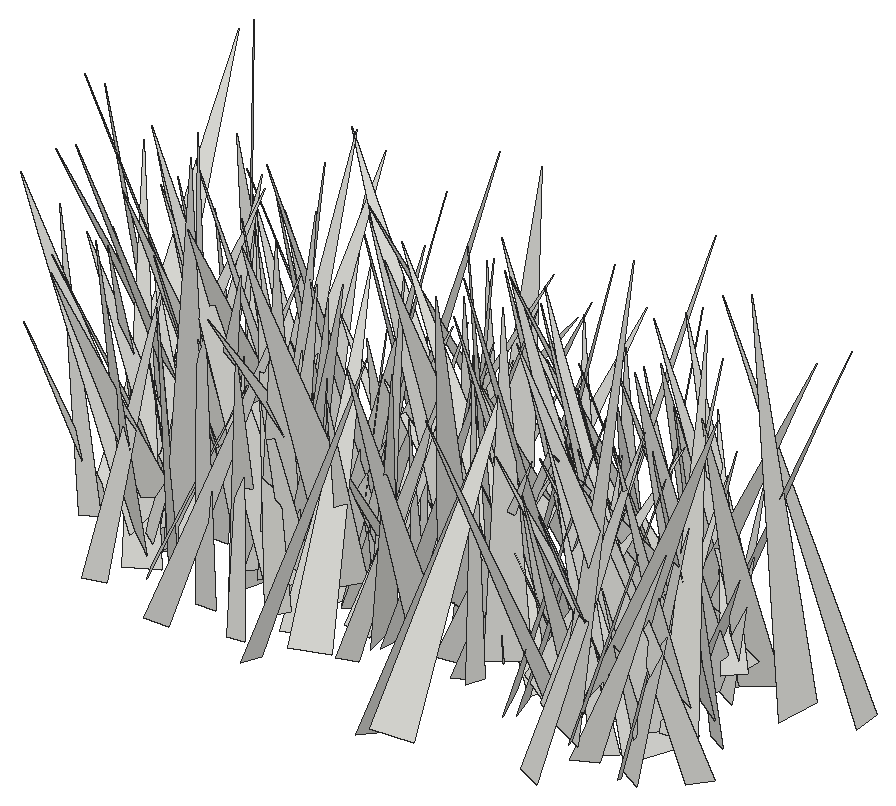
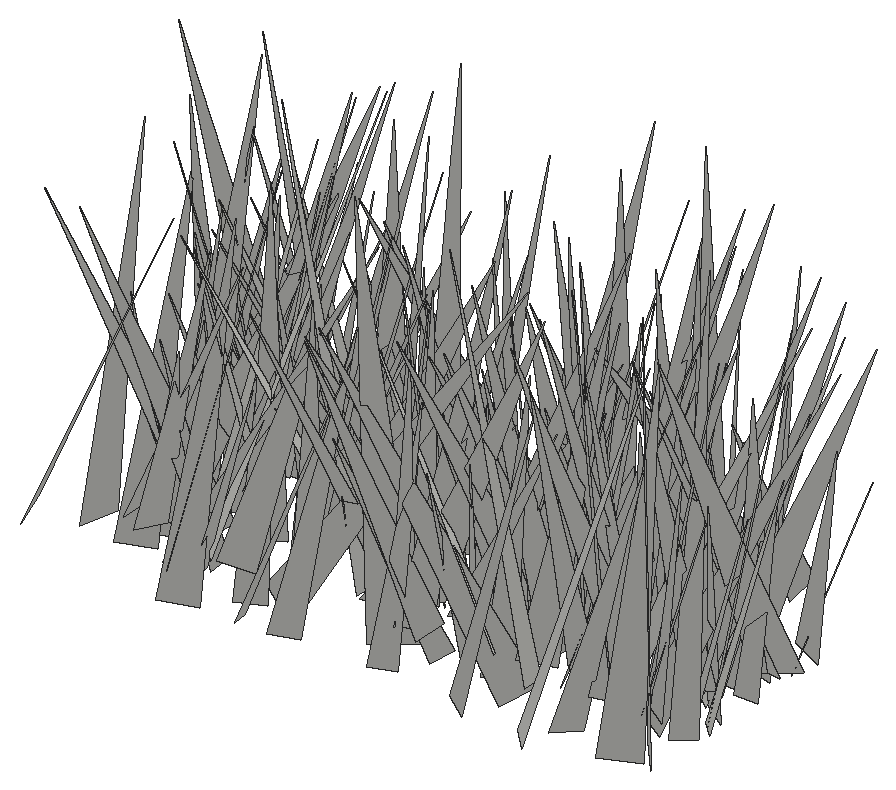
# SketchUp Ruby script. Lengths in inches.
U = 1.inch
M = Sketchup.active_model
def pt(a) = Geom::Point3d.new(a.map { |v| v * U })
def face(e, loops, mat)
  f = e.add_face(loops[0].map { |a| pt(a) })
  loops[1..].each { |l| e.add_face(l.map { |a| pt(a) }).erase! }
  f.material = f.back_material = mat if mat
  f
end
# faces: each face lists its corners as indices into pts; further lists are holes
def faces(e, pts, list, mat = nil) = list.each { |f| face(e, (f[0].is_a?(Array) ? f : [f]).map { |l| l.map { |i| pts[i] } }, mat) }
# xy, xz, yz: faces in a plane at the given z, y or x. An outline is a flat list of corners, or four numbers for a rectangle; further outlines are holes
def ring(l) = l.size == 4 ? [[l[0], l[1]], [l[2], l[1]], [l[2], l[3]], [l[0], l[3]]] : l.each_slice(2).to_a
def flat(e, list, mat, &to3) = list.each { |f| face(e, (f[0].is_a?(Array) ? f : [f]).map { |l| ring(l).map { |u, v| to3.(u, v) } }, mat) }
def xy(e, z, list, mat = nil) = flat(e, list, mat) { |x, y| [x, y, z] }
def xz(e, y, list, mat = nil) = flat(e, list, mat) { |x, z| [x, y, z] }
def yz(e, x, list, mat = nil) = flat(e, list, mat) { |y, z| [x, y, z] }
def lines(e, pts, list) = list.each { |a, b| e.add_line(pt(pts[a]), pt(pts[b])) }
# prism: a flat outline (further loops are holes) pulled along v
def prism(e, loops, v, mat = nil)
  f = face(e, loops, mat); d = Geom::Vector3d.new(v.map { |x| x * U })
  f.pushpull(f.normal.samedirection?(d) ? d.length : -d.length)
end
def box(e, o, s, mat = nil) = prism(e, [[o, [o[0] + s[0], o[1], o[2]], [o[0] + s[0], o[1] + s[1], o[2]], [o[0], o[1] + s[1], o[2]]]], [0, 0, s[2]], mat)
def at(x, y, z, deg = 0) = Geom::Transformation.translation(pt([x, y, z])) * Geom::Transformation.rotation(ORIGIN, Z_AXIS, deg.degrees)
def axes(o, x, y, z) = Geom::Transformation.new([*x, 0, *y, 0, *z, 0, *pt(o).to_a, 1])
def part(name) = M.definitions.add(name)
# library, detail: a bought-in or finely detailed component or shape, given as its bounding box
def library(name, o, s) = part(name).tap { |d| box(d.entities, o, s) }
def detail(e, o, s) = box(e.add_group.entities, o, s)
def put(e, d, t, mat = nil) = e.add_instance(d, t).tap { |i| i.material = mat if mat }
def group(e, t, mat = nil) = e.add_group.tap { |g| g.transformation = t; g.material = mat if mat }.entities
root = M.entities
c1 = part("fur_instance\#9")
p = [[0.8125,0,1.79],[0.67,-0.02,1.48],[0,-0.11,0],[0,0.11,0]]
faces(c1.entities,p,[[0,1,2,3]])
put(root,c1,axes([77.6,147.16,-27.1],[6.21031,-0.46369,2.15458],[0.49806,-5.98034,-2.72263],[-2.14689,-2.7287,5.60092]))
put(root,c1,axes([84.37,145.48,-27.1],[-1.75901,-5.06572,0.78099],[-4.97011,1.48393,-1.5689],[-1.25276,1.22556,5.12778]))
put(root,c1,axes([66.86,146.18,-28.22],[-2.48382,-6.27006,1.58629],[-6.2632,2.75568,1.08533],[1.61318,1.04494,6.65621]))
put(root,c1,axes([80.48,142.09,-28.22],[-3.2571,5.60614,0.8435],[5.30317,3.35677,-1.83235],[2.00417,0.22864,6.21933]))
put(root,c1,axes([85.58,147.03,-27.1],[-2.3415,-4.6423,0.1365],[-4.37976,2.25803,1.66471],[1.54509,-0.63449,4.92568]))
put(root,c1,axes([73.91,143.17,-28.22],[5.46763,0.70402,1.09334],[0.38726,-5.3924,1.5356],[-1.2414,1.41859,5.29457]))
put(root,c1,axes([69.07,144.02,-27.1],[3.47844,1.93474,0.04271],[1.93521,-3.47755,-0.07868],[0.00093,-0.08952,3.97952]))
put(root,c1,axes([67.8125,147.34,-28.22],[2.22572,-6.24997,0.53761],[-6.03536,-2.28904,-1.62473],[-1.71046,-0.05581,6.43243]))
put(root,c1,axes([86.3,144.63,-28.22],[3.70527,-2.55389,0.75103],[-2.66189,-3.54115,1.0909],[0.02774,1.32414,4.36593]))
put(root,c1,axes([68.62,145.87,-28.22],[4.97052,1.68586,2.30908],[2.28367,-5.12743,-1.17229],[-1.72012,-1.9358,5.11604]))
put(root,c1,axes([85.55,142.73,-28.22],[2.91229,5.1803,0.24137],[5.15397,-2.92189,0.52374],[-0.57474,0.04729,5.91968]))
put(root,c1,axes([84.36,146.93,-28.22],[5.01646,-0.03484,2.02413],[0.79085,-4.94522,-2.0451],[-1.86357,-2.19241,4.58078]))
put(root,c1,axes([71.29,141.59,-27.1],[-5.44791,2.04028,1.98238],[0.64646,5.0587,-3.42987],[2.77031,2.83181,4.69878]))
put(root,c1,axes([68.04,142.5,-27.1],[-4.70225,1.57903,0.9136],[0.9953,4.33742,-2.37389],[1.52885,2.03289,4.35536]))
put(root,c1,axes([79.77,141.68,-28.22],[7.02675,2.35333,1.41841],[1.60681,-6.67867,3.12071],[-2.22895,2.60433,6.72121]))
put(root,c1,axes([84.85,144.68,-27.1],[2.54446,5.11145,1.43196],[5.2695,-2.24073,-1.36501],[0.64019,-1.87187,5.54418]))
put(root,c1,axes([72.7,143.875,-28.22],[0.97276,4.45119,0.9772],[4.35496,-1.20232,1.14148],[-1.3425,-0.67498,4.41093]))
put(root,c1,axes([70.92,146.67,-28.22],[4.90376,-2.85552,0.72078],[-2.73926,-4.93651,-0.92072],[-1.08166,-0.44414,5.59939]))
put(root,c1,axes([73.96,148.32,-27.1],[5.79186,-5.56058,1.06137],[-5.14067,-5.80215,-2.34538],[-2.37068,-1.00358,7.67886]))
put(root,c1,axes([88.27,146.18,-27.1],[1.0703,-6.74535,2.51722],[-6.58595,-1.94546,-2.41292],[-2.90886,1.9228,6.3893]))
put(root,c1,axes([68.65,146.46,-27.1],[7.59105,-2.36712,2.02897],[-2.18853,-7.84946,-0.96967],[-2.22043,-0.35586,7.89221]))
put(root,c1,axes([85.88,146.02,-27.1],[6.5822,-3.48627,0.04021],[-3.46978,-6.5418,0.80411],[0.34104,0.72931,7.40492]))
put(root,c1,axes([76.27,146.98,-28.22],[6.47505,-0.26988,1.20187],[0.07267,-6.33614,-1.81428],[-1.22965,-1.79557,6.22153]))
put(root,c1,axes([72.45,146.51,-27.1],[5.8288,-3.89293,1.62458],[-3.86791,-6.0381,-0.59132],[-1.68328,0.3943,6.98428]))
put(root,c1,axes([71.9,143.36,-27.1],[2.76553,6.92914,2.18566],[6.51494,-3.40021,2.53621],[-3.21647,-0.92942,7.01632]))
put(root,c1,axes([86.98,147.06,-28.22],[-5.50457,-1.9976,0.13924],[-1.94432,5.42927,1.02602],[0.47897,-0.91798,5.76524]))
put(root,c1,axes([86.59,145.36,-28.22],[0.57769,-3.84784,2.16026],[-4.16363,-1.197,-1.01866],[-1.46176,1.88882,3.75525]))
put(root,c1,axes([86.07,144,-27.1],[3.67219,7.15908,2.03524],[7.27938,-3.92759,0.68132],[-1.55086,-1.48365,8.01705]))
put(root,c1,axes([67.41,146.14,-27.1],[-3.27496,5.22829,1.96451],[5.47571,2.5569,2.32348],[-1.10043,-2.83671,5.71505]))
put(root,c1,axes([86.4,143.85,-27.1],[4.4489,2.71988,0.66857],[2.4928,-4.41728,1.38241],[-1.27698,0.85286,5.02786]))
put(root,c1,axes([70.7,148.35,-27.1],[0.98136,-7.62341,0.77855],[-7.49654,-1.11781,-1.49599],[-1.58884,0.56543,7.53933]))
put(root,c1,axes([78.21,148.41,-27.1],[0.34985,-8.1007,0.677],[-7.9597,-0.20383,1.67442],[1.6501,0.73429,7.93347]))
put(root,c1,axes([73.08,146.07,-27.1],[-8.06314,0.9505,0.88883],[1.02226,8.07835,0.63476],[0.80526,-0.7379,8.09412]))
put(root,c1,axes([88.92,146.52,-27.1],[-1.01611,-5.1437,1.43202],[-5.3112,0.8243,-0.80778],[-0.54728,1.55038,5.1805]))
put(root,c1,axes([73.09,147,-28.22],[3.60801,-2.69307,1.35493],[-2.4926,-3.85347,-1.02171],[-1.69571,-0.06573,4.3848]))
put(root,c1,axes([87.72,145.82,-27.1],[-7.02647,-2.17808,1.10616],[-2.29777,7.03636,-0.74079],[0.82938,1.04138,7.31892]))
put(root,c1,axes([64.94,146.83,-27.1],[-3.14416,-1.79317,0.28571],[-1.75542,3.14785,0.43854],[0.46429,-0.24163,3.59289]))
put(root,c1,axes([82.13,146.03,-28.22],[6.04949,2.12455,0.78775],[2.22415,-5.99674,-0.90711],[-0.43293,-1.1207,6.34722]))
put(root,c1,axes([90.05,145.83,-28.22],[-1.48445,-5.73193,2.26963],[-5.6541,0.33538,-2.85107],[-2.45713,2.69116,5.18942]))
put(root,c1,axes([67.28,148.54,-28.22],[-4.43936,-4.76816,0.23664],[-4.66276,4.39992,1.18262],[1.02469,-0.63608,6.40661]))
put(root,c1,axes([82.59,146.125,-28.22],[4.18181,1.0835,0.53294],[1.13424,-4.18373,-0.39425],[-0.41412,-0.51766,4.30187]))
put(root,c1,axes([81.59,146.6,-27.1],[4.24659,-4.94069,2.32668],[-5.22174,-4.53655,-0.10277],[-1.59916,1.69313,6.51409]))
put(root,c1,axes([73.99,144.41,-27.1],[-6.21207,0.31771,0.7174],[0.09871,5.99609,-1.80072],[0.77837,1.77522,5.95384]))
put(root,c1,axes([72.21,147.16,-28.22],[-7.46338,-1.41905,1.28497],[-1.31215,7.55774,0.72509],[1.39396,-0.48353,7.56241]))
put(root,c1,axes([87.75,146.16,-28.22],[-6.89397,4.20656,1.53795],[4.42912,6.82252,1.19307],[0.66584,-1.82904,7.9874]))
put(root,c1,axes([81.63,144.92,-27.1],[-5.20455,-0.25594,1.25726],[-0.61037,5.11409,-1.48563],[1.12857,1.58561,4.99457]))
put(root,c1,axes([83.66,147.67,-27.1],[-3.27464,-6.78559,1.40651],[-6.92909,3.22889,-0.5548],[0.10135,1.50857,7.51397]))
put(root,c1,axes([86.16,147.91,-28.22],[-3.67064,-4.64361,1.03864],[-4.58105,3.8034,0.81465],[1.28682,0.29416,5.86285]))
put(root,c1,axes([74.65,147.45,-27.1],[2.8154,-3.04723,0.70248],[-2.99803,-2.89898,-0.55973],[-0.88933,0.126,4.11081]))
put(root,c1,axes([72.54,151.18,-28.22],[-6.33754,-5.19611,0.8236],[-4.02771,5.62162,4.47406],[3.3846,-3.03975,6.86635]))
put(root,c1,axes([86.71,146.34,-27.1],[-8.26176,0.40654,0.83522],[0.41692,8.30295,0.08258],[0.83009,-0.12394,8.27135]))
put(root,c1,axes([72.48,147.22,-27.1],[6.13982,-1.63324,0.91897],[-1.58888,-6.20592,-0.4139],[-0.99371,-0.16841,6.33984]))
put(root,c1,axes([68.72,149.125,-28.22],[-3.15588,-6.30761,0.73503],[-6.08642,3.23856,1.65924],[1.81157,-0.10755,6.85511]))
put(root,c1,axes([78.95,147.05,-28.22],[3.19208,-3.97574,0.46961],[-3.91795,-2.97897,1.41133],[0.82265,1.2392,4.89939]))
put(root,c1,axes([67.33,146.47,-27.1],[2.36922,2.94645,1.17355],[3.15581,-2.33594,-0.5062],[-0.31572,-1.23846,3.7468]))
put(root,c1,axes([67.6,145.81,-27.1],[2.29816,3.3477,0.63042],[3.39972,-2.30202,-0.16916],[-0.21536,-0.61617,4.05709]))
put(root,c1,axes([72.42,147.91,-27.1],[-0.76172,-5.93829,1.58025],[-5.83151,1.20063,1.7008],[1.93753,1.27903,5.74028]))
put(root,c1,axes([73.89,145.35,-28.22],[-2.71251,3.20119,0.88639],[3.03008,2.85354,-1.03292],[1.36084,0.02704,4.06674]))
put(root,c1,axes([72.01,147.28,-27.1],[0.25447,-5.59234,1.88155],[-5.79418,0.11887,1.13692],[1.11444,1.89496,5.48146]))
put(root,c1,axes([67.75,148.5,-28.22],[2.61473,-6.42495,0.46001],[-6.33227,-2.47287,1.45453],[1.18065,0.96609,6.78241]))
put(root,c1,axes([65.3125,145.67,-27.1],[0.45308,4.94253,1.25959],[4.74966,-0.86975,1.70432],[-1.859,-1.01755,4.66145]))
put(root,c1,axes([87.91,144.38,-28.22],[3.78632,3.0497,0.88341],[2.42458,-3.66486,2.25998],[-2.05,1.29824,4.30457]))
put(root,c1,axes([75.03,144.73,-28.22],[-3.56616,5.34471,0.77163],[5.27091,3.64619,-0.89538],[1.17426,-0.13507,6.36253]))
put(root,c1,axes([81.02,146.8,-27.1],[3.81307,5.29138,3.34018],[5.75803,-4.49829,0.55278],[-2.44962,-2.33704,6.49867]))
put(root,c1,axes([83.95,147.6,-28.22],[-2.77092,-3.22119,0.17285],[-3.17409,2.68192,-0.90354],[-0.57541,0.71776,4.15182]))
put(root,c1,axes([88.18,144.62,-28.22],[3.93079,5.90323,1.06815],[5.73682,-4.07234,1.39466],[-1.7544,-0.09002,6.95371]))
put(root,c1,axes([68.27,148.74,-27.1],[-3.1759,-6.57357,0.78945],[-6.61199,3.10387,-0.75436],[-0.34161,1.03711,7.26148]))
put(root,c1,axes([69.45,145.89,-27.1],[-1.35626,4.67986,0.4324],[4.48876,1.15652,1.56235],[-1.3925,-0.82998,4.61514]))
put(root,c1,axes([88.56,148.07,-27.1],[-3.05463,-4.97038,1.37571],[-5.09206,3.16016,0.11108],[0.81742,1.11209,5.83293]))
put(root,c1,axes([82.23,148.48,-27.1],[-5.80555,-2.80529,1.19859],[-2.69051,5.92298,0.83076],[1.43785,-0.24369,6.39405]))
put(root,c1,axes([83.24,145.84,-27.1],[2.06268,4.77096,0.10661],[4.57909,-1.94603,-1.50762],[1.34363,-0.69206,4.97431]))
put(root,c1,axes([88.98,146.08,-27.1],[-0.28002,6.79198,1.74012],[7.00527,0.19856,0.35229],[-0.29175,-1.75129,6.78861]))
put(root,c1,axes([72.28,148.1875,-27.1],[-3.33376,-1.76985,1.3611],[-1.54667,3.5947,0.88593],[1.61021,-0.21143,3.66899]))
put(root,c1,axes([71.61,146.21,-27.1],[0.20171,6.63601,2.13173],[6.14884,-1.17367,3.07178],[-3.28217,-1.79094,5.8857]))
put(root,c1,axes([76.74,146.88,-28.22],[6.15775,0.09619,0.89999],[0.03195,-6.20791,0.44493],[-0.90455,0.43558,6.14241]))
put(root,c1,axes([67.01,148.05,-28.22],[-2.6203,-2.567,1.06702],[-2.53846,2.80716,0.51965],[1.13325,0.35259,3.63117]))
put(root,c1,axes([82.67,147.8125,-28.22],[-0.62514,-3.66803,1.11265],[-3.82799,0.53943,-0.37244],[-0.19721,1.15663,3.70223]))
put(root,c1,axes([76.65,148.99,-28.22],[-1.76635,-5.02439,0.02248],[-4.81779,1.68692,-1.51928],[-1.42615,0.52421,5.10454]))
put(root,c1,axes([72.72,147.5,-28.22],[-6.09908,-2.25868,1.59557],[-2.41433,6.23322,-0.4051],[1.3485,0.94419,6.49124]))
put(root,c1,axes([67.51,148.23,-28.22],[-4.26864,3.3889,1.68719],[3.78174,3.93314,1.66776],[0.17248,-2.36607,5.18889]))
put(root,c1,axes([71.43,147.67,-28.22],[2.82184,-3.33686,1.43593],[-3.57868,-2.86589,0.37288],[-0.62414,1.34588,4.35412]))
put(root,c1,axes([64.98,149.18,-27.1],[-0.80762,-5.18,0.70533],[-5.16495,0.90095,0.70267],[0.80822,0.5814,5.19528]))
put(root,c1,axes([85.72,148.88,-27.1],[-4.15133,-1.53142,0.10873],[-1.49707,4.10736,0.69206],[0.34034,-0.61232,4.37033]))
put(root,c1,axes([67.5,145.6,-28.22],[-1.06159,6.87885,0.56166],[6.76624,0.92524,1.45707],[-1.36093,-0.76575,6.80607]))
put(root,c1,axes([84.23,147.12,-28.22],[0.52075,4.40411,1.27547],[4.58416,-0.47433,-0.2338],[0.09203,-1.29345,4.42863]))
put(root,c1,axes([86.7,150.61,-28.22],[5.51708,-5.76072,0.82028],[-5.55442,-5.55067,-1.6234],[-1.73412,-0.54876,7.80952]))
put(root,c1,axes([76.29,145.05,-28.22],[5.42,0.95377,1.93695],[-0.10115,-5.11614,2.80228],[-2.15667,2.63692,4.73638]))
put(root,c1,axes([85.24,149.54,-28.22],[-6.08575,-1.31512,1.93305],[-0.80976,6.24223,1.69745],[2.19329,-1.34444,5.99037]))
put(root,c1,axes([74.31,147.95,-27.1],[3.95435,2.54343,1.52337],[2.80761,-4.0284,-0.56212],[-0.95239,-1.31514,4.66797]))
put(root,c1,axes([68.22,151.98,-27.1],[7.18044,-3.7228,0.21814],[-3.29243,-6.55088,-3.42221],[-1.75122,-2.94828,7.32847]))
put(root,c1,axes([75.4,146.68,-28.22],[-0.65991,4.20046,0.70673],[4.09857,0.8209,-1.05196],[1.15975,-0.51096,4.1198]))
put(root,c1,axes([75.35,147.9,-28.22],[-2.04646,-5.42862,2.85461],[-5.95901,2.47232,0.42963],[1.45222,2.49488,5.78561]))
put(root,c1,axes([86.55,151.64,-27.1],[3.78174,-4.82109,0.17581],[-4.12071,-3.34423,-3.06777],[-2.50869,-1.77444,5.30408]))
put(root,c1,axes([73.84,148.1,-28.22],[-3.54918,2.04608,0.76374],[2.14815,3.53344,0.51649],[0.39398,-0.83357,4.06404]))
put(root,c1,axes([71.15,148.3,-27.1],[5.93404,-1.49093,1.99542],[-1.59561,-6.23409,0.08712],[-1.91274,0.57506,6.11785]))
put(root,c1,axes([82.6,147.7,-28.22],[-4.85114,5.94494,0.47809],[5.69058,4.42924,2.66526],[-1.78556,-2.03568,7.19529]))
put(root,c1,axes([76.52,149.1,-28.22],[5.2345,0.58731,0.96902],[0.7581,-5.21929,-0.93179],[-0.84215,-1.04786,5.18428]))
put(root,c1,axes([88.82,148.21,-28.22],[-3.42512,-4.29344,1.99666],[-4.721,3.28594,-1.03273],[0.36395,2.21827,5.39431]))
put(root,c1,axes([75.99,149.125,-28.22],[1.30343,6.50873,4.51627],[7.0846,-3.00591,2.28737],[-3.54523,-3.61388,6.23141]))
put(root,c1,axes([85.39,150.96,-27.1],[-4.26482,-5.03014,0.77761],[-4.82923,4.31941,1.45497],[1.60794,-0.36894,6.43227]))
put(root,c1,axes([75.97,149.14,-28.22],[-3.40135,-0.48301,1.73948],[-0.24917,3.80046,0.56808],[1.78802,-0.38922,3.38818]))
put(root,c1,axes([65.44,147.44,-27.1],[2.30365,5.6713,0.71156],[5.64313,-2.13475,-1.25489],[0.90837,-1.12069,5.9913]))
put(root,c1,axes([83.89,150.62,-27.1],[-3.75985,-4.2409,1.14983],[-3.97997,3.92819,1.47409],[1.86202,-0.16705,5.47255]))
put(root,c1,axes([82.05,149.6,-27.1],[-5.02334,-0.16728,0.55191],[-0.071,4.98153,0.86367],[0.57231,-0.85028,4.95137]))
put(root,c1,axes([74.08,148.16,-28.22],[4.7492,-0.22527,1.39473],[-0.44396,-4.88167,0.72329],[-1.34124,0.81823,4.6992]))
put(root,c1,axes([86.6,147.45,-28.22],[0.96438,4.41888,0.40988],[4.43511,-0.94495,-0.24768],[0.15571,-0.45288,4.5161]))
put(root,c1,axes([69.41,149.18,-27.1],[-5.59942,-5.49473,0.70955],[-5.42162,5.22657,-2.3104],[-1.14084,2.13071,7.49717]))
put(root,c1,axes([66.49,149.03,-28.22],[-6.58446,-3.61184,1.85584],[-3.84727,6.67992,-0.64953],[1.29924,1.4758,7.48189]))
put(root,c1,axes([67.83,150.64,-28.22],[-2.71774,-6.73125,0.47193],[-6.54696,2.5072,-1.9416],[-1.63394,1.15011,6.99472]))
put(root,c1,axes([78,149.14,-27.1],[-6.68615,-0.01766,0.93467],[0.01232,6.74773,0.2156],[0.93476,-0.21523,6.6827]))
put(root,c1,axes([79.89,146.35,-28.22],[5.42222,1.22065,1.50489],[0.3801,-5.05507,2.73075],[-1.90005,2.47215,4.84081]))
put(root,c1,axes([64.89,152.46,-27.1],[-1.50636,-7.45489,0.25307],[-6.77182,1.47502,3.14252],[3.12761,-0.39686,6.92598]))
put(root,c1,axes([84.23,152.44,-27.1],[-5.99255,-5.60768,0.41861],[-5.37957,5.89507,1.95969],[1.63755,-1.155,7.96972]))
put(root,c1,axes([85.02,149.47,-27.1],[3.32524,-3.2763,0.88677],[-3.39381,-3.22791,0.80025],[-0.05063,1.1934,4.59902]))
put(root,c1,axes([76.13,152.2,-27.1],[6.61822,-2.56323,1.80089],[-1.74555,-6.51281,-2.85492],[-2.60123,-2.15113,6.49773]))
put(root,c1,axes([81.86,150.76,-27.1],[-0.45629,-4.37673,0.42276],[-4.25435,0.54685,1.06962],[1.11127,0.29645,4.26847]))
put(root,c1,axes([72.79,149.47,-27.1],[-3.17,-4.98135,1.74667],[-5.27871,2.99065,-1.05117],[-0.00204,2.03858,5.81015]))
put(root,c1,axes([72.33,150.6875,-27.1],[-2.39227,-3.29447,0.41561],[-3.24315,2.42809,0.57931],[0.71291,-0.00928,4.03]))
put(root,c1,axes([77.61,149.24,-28.22],[3.62695,2.69385,0.06353],[2.59465,-3.4627,-1.30122],[0.7271,-1.08099,4.32648]))
put(root,c1,axes([71.66,149.92,-28.22],[-6.57116,-2.81105,0.67584],[-2.85659,6.57143,-0.44162],[0.44572,0.67315,7.13352]))
put(root,c1,axes([72.68,148.99,-28.22],[6.40804,-1.16691,1.44574],[-1.35043,-6.49108,0.74636],[-1.27601,1.00946,6.47052]))
put(root,c1,axes([72.91,148.82,-27.1],[4.25693,-2.37845,0.80532],[-2.50825,-3.95225,1.586],[0.11926,1.77474,4.61119]))
put(root,c1,axes([68.28,150.23,-28.22],[-5.55068,-3.03255,1.58004],[-3.06213,5.7489,0.27653],[1.52193,0.50669,6.31901]))
put(root,c1,axes([69.15,149.35,-28.22],[1.6675,5.06938,1.93589],[5.41393,-1.41673,-0.95346],[0.36831,-2.12629,5.25072]))
put(root,c1,axes([78.07,148.34,-28.22],[3.82909,4.88275,1.88302],[4.81565,-4.20088,1.10051],[-2.04855,-0.74856,6.10673]))
put(root,c1,axes([83.29,150.68,-27.1],[3.25628,-4.96201,1.27437],[-5.08219,-3.31911,0.06246],[-0.64574,1.10043,5.93473]))
put(root,c1,axes([79.33,150.15,-28.22],[-3.75948,2.94392,0.27379],[2.73653,3.29698,2.12525],[-1.1194,-1.82718,4.27594]))
put(root,c1,axes([69.7,148.4,-27.1],[-4.60941,2.24833,0.68921],[2.12734,4.63308,-0.88638],[1.00221,0.50623,5.05134]))
put(root,c1,axes([87.64,151.94,-28.22],[3.11864,-5.68803,0.55795],[-5.6529,-3.16353,-0.65398],[-0.84244,0.17118,6.45383]))
put(root,c1,axes([78.83,151.27,-27.1],[7.66511,2.45698,1.17946],[2.70747,-7.26796,-2.45522],[-0.3122,-2.70587,7.66567]))
put(root,c1,axes([73.84,149.38,-28.22],[0.15011,3.96157,1.30257],[3.86973,0.35348,-1.52101],[1.55431,-1.26265,3.66102]))
put(root,c1,axes([77.63,151.53,-27.1],[-4.01189,-2.17426,1.82805],[-1.57492,4.33524,1.69992],[2.36407,-0.80168,4.23473]))
put(root,c1,axes([66.4,149.02,-28.22],[1.72426,4.07776,1.35625],[4.04188,-2.03524,0.98061],[-1.4597,-0.81871,4.31736]))
put(root,c1,axes([85.99,152.26,-28.22],[-5.52668,-3.91053,1.22579],[-3.5737,5.60606,1.77193],[2.00587,-0.78663,6.53427]))
put(root,c1,axes([82.41,152.64,-28.22],[0.16634,-6.6201,0.01552],[-6.42128,-0.15757,1.61124],[1.61035,0.05552,6.42319]))
put(root,c1,axes([71.61,151.54,-27.1],[3.35042,-5.0359,1.55374],[-4.92978,-3.64566,-1.18576],[-1.86322,0.59037,5.93123]))
put(root,c1,axes([73.25,151.46,-28.22],[3.51488,-3.51732,0.75482],[-3.443,-3.59499,-0.71937],[-1.04262,0.01399,4.9202]))
put(root,c1,axes([76.94,150.69,-27.1],[0.54293,-5.17192,1.62827],[-5.42158,-0.49338,0.24063],[0.08095,1.64396,5.19477]))
put(root,c1,axes([70.75,147.87,-27.1],[0.90222,6.95991,0.72818],[6.98982,-0.93156,0.24337],[-0.33621,-0.69025,7.01392]))
put(root,c1,axes([66.5,149.64,-27.1],[-0.43128,5.47544,2.09207],[5.72554,0.84273,-1.02531],[1.25517,-1.9628,5.39585]))
put(root,c1,axes([64.72,151.46,-27.1],[-3.11694,-3.18155,0.61605],[-3.14817,3.17551,0.47138],[0.76862,0.10457,4.42892]))
put(root,c1,axes([82.99,152.63,-27.1],[2.63198,-5.20128,0.6124],[-4.94839,-2.69423,-1.6156],[-1.71515,-0.20845,5.60093]))
put(root,c1,axes([86,151.77,-28.22],[-7.00038,0.48524,0.02911],[0.47648,6.76613,1.79834],[-0.09628,-1.796,6.78283]))
put(root,c1,axes([65.25,147.24,-27.1],[-3.2389,7.2108,0.31573],[7.08918,3.2432,-1.34571],[1.35602,0.26802,7.78942]))
put(root,c1,axes([75.41,150.67,-27.1],[-3.7614,2.09395,0.36046],[2.10674,3.58022,1.1859],[-0.27609,-1.20834,4.13841]))
put(root,c1,axes([81.25,151.44,-28.22],[-6.2182,-2.45212,1.53392],[-2.39925,6.40419,0.51167],[1.61537,0.0727,6.66461]))
put(root,c1,axes([65.89,150.62,-27.1],[-2.9488,-2.48385,0.84804],[-2.61567,2.88641,-0.64107],[0.2167,1.04076,3.80183]))
put(root,c1,axes([85.24,148.4375,-27.1],[4.44395,3.96646,1.43413],[3.47391,-4.62357,2.02305],[-2.39195,0.65422,5.60257]))
put(root,c1,axes([83.43,146.66,-28.22],[5.15692,6.28398,0.1894],[5.87834,-4.90651,2.73667],[-2.22922,1.59869,7.6546]))
put(root,c1,axes([87.12,150.6875,-28.22],[1.48907,3.83094,1.46531],[4.09712,-1.31638,-0.722],[0.19182,-1.62223,4.04625]))
put(root,c1,axes([75.77,149.54,-28.22],[1.76698,3.75792,1.11012],[3.4505,-2.06932,1.51278],[-1.85698,-0.26926,3.86726]))
put(root,c1,axes([67.03,151.77,-27.1],[-3.51503,-1.89548,0.64915],[-1.82323,3.56963,0.55065],[0.83071,-0.18586,3.95538]))
put(root,c1,axes([82.14,150.02,-28.22],[-5.1029,2.41175,1.4356],[2.37658,5.2976,-0.4521],[1.4931,-0.1897,5.62599]))
put(root,c1,axes([68.2,151.92,-28.22],[5.45903,4.38742,2.52703],[5.0114,-5.21201,-1.77686],[-0.72192,-3.00365,6.77446]))
put(root,c1,axes([81.63,152.15,-28.22],[-3.41379,-7.32141,0.63154],[-6.65452,2.7845,-3.69049],[-3.11756,2.07349,7.18591]))
put(root,c1,axes([89.65,151.3,-28.22],[-7.15931,0.95304,2.49675],[1.12982,7.54938,0.35801],[2.42189,-0.70454,7.21359]))
put(root,c1,axes([69.58,149.4,-27.1],[-0.94911,6.39885,1.08787],[6.32075,1.1611,-1.31509],[1.4754,-0.85797,6.33377]))
put(root,c1,axes([86.53,149.51,-28.22],[6.67299,1.88656,0.54903],[1.75109,-6.59185,1.3677],[-0.89119,1.17381,6.79833]))
put(root,c1,axes([73.15,151.68,-27.1],[5.8637,3.4963,0.04079],[3.31459,-5.53283,-2.23832],[1.11324,-1.94227,6.44958]))
put(root,c1,axes([74.34,147.76,-28.22],[-6.96158,0.42843,3.50828],[-1.43896,6.73486,-3.67782],[3.22816,3.92599,5.92628]))
put(root,c1,axes([77.11,150.625,-27.1],[-5.54363,5.04114,0.10568],[4.92423,5.3789,1.72499],[-1.08457,-1.34553,7.29173]))
put(root,c1,axes([70.92,152.61,-27.1],[6.83601,2.20523,1.02382],[2.40175,-6.59991,-1.82073],[-0.37792,-2.05437,6.94831]))
put(root,c1,axes([66.55,151.79,-27.1],[-2.19445,-3.56039,1.55722],[-3.85398,2.22319,-0.34801],[0.4981,1.5159,4.16783]))
put(root,c1,axes([84.75,151.27,-28.22],[4.10361,0.18993,0.89205],[0.09258,-4.17709,0.46346],[-0.90734,0.43277,4.08178]))
put(root,c1,axes([80.24,153.64,-28.22],[3.73723,-3.51523,0.8829],[-3.22394,-3.80362,-1.49732],[-1.65607,-0.52811,4.90732]))
put(root,c1,axes([78,150.08,-28.22],[1.18506,6.07091,0.5983],[5.8889,-0.9794,-1.72625],[1.5921,-0.89616,5.93973]))
put(root,c1,axes([87.76,150.43,-27.1],[-1.23895,4.11427,0.01816],[3.97981,1.19363,1.09497],[-1.04341,-0.33255,4.15491]))
put(root,c1,axes([77.2,151.79,-28.22],[-3.47226,6.33449,3.63746],[6.89094,4.17667,-0.69553],[2.42317,-2.80055,7.19017]))
put(root,c1,axes([87.85,151.61,-27.1],[-5.92651,0.06077,0.05927],[0.05827,5.92175,-0.24529],[0.06173,0.24468,5.92174]))
put(root,c1,axes([74.625,151.36,-28.22],[3.22488,1.438,0.95498],[1.40641,-3.36208,0.31327],[-1.00092,-0.09099,3.51704]))
put(root,c1,axes([84.82,151.23,-27.1],[5.89255,-1.31891,0.46121],[-1.38894,-5.74659,1.31223],[-0.15186,1.38261,5.89404]))
put(root,c1,axes([70.07,151.08,-27.1],[-0.06431,5.36711,1.48252],[5.54585,0.19413,-0.46222],[0.49719,-1.47116,5.34755]))
put(root,c1,axes([84.21,154.0625,-28.22],[3.11347,-5.57932,0.56956],[-5.54553,-3.1599,-0.63956],[-0.83685,0.18197,6.35716]))
put(root,c1,axes([82.07,153.59,-28.22],[-4.41173,-1.92667,0.46008],[-1.77307,4.34177,1.17998],[0.88316,-0.90777,4.66723]))
put(root,c1,axes([71.99,151.97,-28.22],[4.62991,-4.98565,0.093],[-4.3743,-3.99984,3.34189],[2.39393,2.33366,5.92659]))
put(root,c1,axes([66.88,153.25,-28.22],[3.62749,-5.55241,1.8821],[-5.65778,-3.89547,-0.58748],[-1.5366,1.23544,6.60627]))
put(root,c1,axes([76.99,151.7,-27.1],[-4.7956,1.01448,1.55419],[0.95492,5.04106,-0.34401],[1.59148,0.0322,4.88965]))
put(root,c1,axes([70.24,154.15,-28.22],[-4.85913,-4.7221,0.69622],[-4.68141,4.90862,0.61965],[0.93132,0.03646,6.74725]))
put(root,c1,axes([75.47,151.54,-28.22],[3.57113,-2.0967,0.79041],[-2.23153,-3.1932,1.61171],[0.20288,1.78359,3.81464]))
put(root,c1,axes([86.79,152.22,-27.1],[-5.29366,2.0126,1.17564],[2.12712,5.36423,0.39489],[0.95291,-0.79376,5.64955]))
put(root,c1,axes([76.48,153.33,-28.22],[2.46831,-3.73303,1.12427],[-3.72872,-2.64901,-0.60947],[-1.13849,0.58247,4.43358]))
put(root,c1,axes([91.73,152.1875,-28.22],[-7.1325,-1.97369,0.04131],[-1.9512,7.0246,-1.27181],[-0.29997,1.23662,7.29044]))
put(root,c1,axes([69.39,152.82,-28.22],[-4.78062,2.36193,1.12593],[2.54726,4.73726,0.87783],[0.59826,-1.2963,5.25951]))
put(root,c1,axes([75.52,152.1,-27.1],[5.25696,-1.00652,0.21452],[-1.02902,-5.15697,1.02054],[-0.01477,1.04274,5.25426]))
put(root,c1,axes([66.35,152.39,-28.22],[-5.7343,-4.84539,3.53032],[-5.45543,6.24306,-0.29262],[2.4858,2.5238,7.50162]))
put(root,c1,axes([73.16,153.74,-28.22],[-3.14093,-4.54056,1.19879],[-4.68857,3.11384,-0.49041],[0.26658,1.26749,5.49924]))
put(root,c1,axes([84.79,152.35,-28.22],[-4.76571,-0.2474,0.30777],[-0.30187,4.68534,-0.90794],[0.25457,0.92426,4.68496]))
